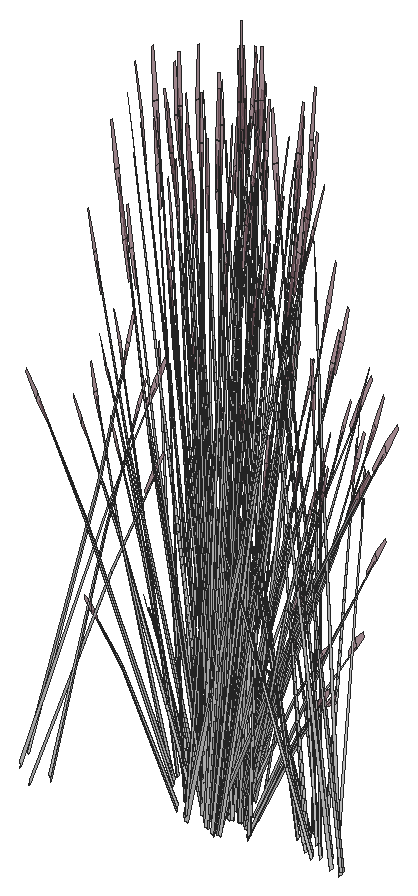
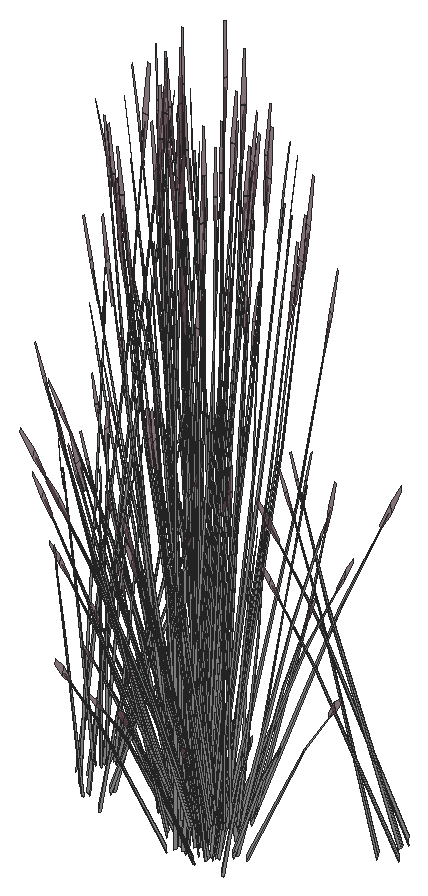
# SketchUp Ruby script. Lengths in inches.
U = 1.inch
M = Sketchup.active_model
def pt(a) = Geom::Point3d.new(a.map { |v| v * U })
def face(e, loops, mat)
  f = e.add_face(loops[0].map { |a| pt(a) })
  loops[1..].each { |l| e.add_face(l.map { |a| pt(a) }).erase! }
  f.material = f.back_material = mat if mat
  f
end
# faces: each face lists its corners as indices into pts; further lists are holes
def faces(e, pts, list, mat = nil) = list.each { |f| face(e, (f[0].is_a?(Array) ? f : [f]).map { |l| l.map { |i| pts[i] } }, mat) }
# xy, xz, yz: faces in a plane at the given z, y or x. An outline is a flat list of corners, or four numbers for a rectangle; further outlines are holes
def ring(l) = l.size == 4 ? [[l[0], l[1]], [l[2], l[1]], [l[2], l[3]], [l[0], l[3]]] : l.each_slice(2).to_a
def flat(e, list, mat, &to3) = list.each { |f| face(e, (f[0].is_a?(Array) ? f : [f]).map { |l| ring(l).map { |u, v| to3.(u, v) } }, mat) }
def xy(e, z, list, mat = nil) = flat(e, list, mat) { |x, y| [x, y, z] }
def xz(e, y, list, mat = nil) = flat(e, list, mat) { |x, z| [x, y, z] }
def yz(e, x, list, mat = nil) = flat(e, list, mat) { |y, z| [x, y, z] }
def lines(e, pts, list) = list.each { |a, b| e.add_line(pt(pts[a]), pt(pts[b])) }
# prism: a flat outline (further loops are holes) pulled along v
def prism(e, loops, v, mat = nil)
  f = face(e, loops, mat); d = Geom::Vector3d.new(v.map { |x| x * U })
  f.pushpull(f.normal.samedirection?(d) ? d.length : -d.length)
end
def box(e, o, s, mat = nil) = prism(e, [[o, [o[0] + s[0], o[1], o[2]], [o[0] + s[0], o[1] + s[1], o[2]], [o[0], o[1] + s[1], o[2]]]], [0, 0, s[2]], mat)
def at(x, y, z, deg = 0) = Geom::Transformation.translation(pt([x, y, z])) * Geom::Transformation.rotation(ORIGIN, Z_AXIS, deg.degrees)
def axes(o, x, y, z) = Geom::Transformation.new([*x, 0, *y, 0, *z, 0, *pt(o).to_a, 1])
def part(name) = M.definitions.add(name)
# library, detail: a bought-in or finely detailed component or shape, given as its bounding box
def library(name, o, s) = part(name).tap { |d| box(d.entities, o, s) }
def detail(e, o, s) = box(e.add_group.entities, o, s)
def put(e, d, t, mat = nil) = e.add_instance(d, t).tap { |i| i.material = mat if mat }
def group(e, t, mat = nil) = e.add_group.tap { |g| g.transformation = t; g.material = mat if mat }.entities
root = M.entities
M.materials.add("LightPink_Translucent").color = [144, 107, 117]
M.materials["LightPink_Translucent"].alpha = 0.75
M.materials.add("[_0053_Ivory_]").color = [200, 200, 200]
c1 = part("blade")
p = [[2.15,0.21,22],[0,0.17,0],[0.09,0.45,0],[2.18,0.31,22],[2.29,0.31,22],[0.38,0.45,0],
  [2.48,0.24,33],[2.49,0.24,33],[2.48,0.22,33]]
faces(c1.entities,p,[[0,1,2,3],[4,5,2,3],[6,3,4,7],[8,0,3,6]])
c2 = part("seeds")
p = [[0.3,-0.1,1.38],[-0.01,-0.03,1.59],[-0.01,-0.03,0.03],[0.14,-0.07,-0.07],[0.29,-0.03,3],[0.15,0.01,3.11]]
faces(c2.entities,p,[[0,1,2,3],[1,0,4,5]],"LightPink_Translucent")
c3 = part("blade with seeds")
put(c3.entities,c1,at(0,0,0))
put(c3.entities,c2,axes([2.4,0.25,30.99],[1.5799,-0.05474,1.17369],[-0.12525,1.92788,0.29478],[-0.07173,-0.02425,1.56792]))
put(root,c3,axes([443.95,105.24,129.13],[0,0.62885,0.49651],[-0.67951,0,0],[0,-0.14322,1.57504]),"[_0053_Ivory_]")
put(root,c3,axes([458.43,104.23,129.32],[-0.61322,0.4175,-0.29095],[-0.40778,-0.58992,-0.50002],[-0.1513,-0.05991,1.59708]),"[_0053_Ivory_]")
put(root,c3,axes([448.72,105.38,131.33],[0.16454,-0.57202,-0.51099],[0.56413,0.19607,-0.3958],[0.22713,-0.05245,0.97773]),"[_0053_Ivory_]")
put(root,c3,axes([447.83,103.05,129.03],[0.37973,-0.63014,0],[0.6353,0.35142,-0.51607],[0.14469,0.08004,1.63711]),"[_0053_Ivory_]")
put(root,c3,axes([443.36,104.3,130.53],[0.25192,-0.01424,1.71376],[-0.16712,0.61729,0.13857],[-0.35901,-0.03818,0.73262]),"[_0053_Ivory_]")
put(root,c3,axes([445.56,105.75,128.86],[-0.36485,-0.52782,-0.44739],[0.55265,-0.37168,0.21531],[-0.11807,-0.06531,1.43643]),"[_0053_Ivory_]")
put(root,c3,axes([445.63,105,129.01],[0.26406,0.70318,0.45755],[-0.7545,0.24452,0.17955],[0.00922,-0.12921,1.58856]),"[_0053_Ivory_]")
put(root,c3,axes([434.7,101.25,129.32],[-0.38947,-0.01972,1.0506],[0.25721,-0.41888,0.58006],[0.15386,0.14882,0.8241]),"[_0053_Ivory_]")
put(root,c3,axes([449.33,105.54,128.64],[-0.39118,0.07547,1.41583],[-0.06226,-0.6007,0.08104],[0.27398,-0.09092,0.80566]),"[_0053_Ivory_]")
put(root,c3,axes([450.04,105.01,128.91],[-0.37654,-0.40212,-0.06488],[0.4124,-0.36845,-0.29416],[0.11685,-0.02594,0.97024]),"[_0053_Ivory_]")
put(root,c3,axes([445.5,105.56,129.37],[-0.29468,0.56664,0.44739],[-0.61229,-0.27271,-0.21531],[0,-0.13062,1.43643]),"[_0053_Ivory_]")
put(root,c3,axes([446.58,105.0625,128.86],[0,-0.72763,0],[0.75945,0,0],[0,0,1.79456]),"[_0053_Ivory_]")
put(root,c3,axes([447.5,103.38,129.13],[-0.56842,-0.31443,0.49651],[0.33976,-0.56381,0],[0.12946,0.07161,1.57504]),"[_0053_Ivory_]")
put(root,c3,axes([448.62,105.59,131.63],[0.53369,-0.27773,-0.71045],[0.29743,0.5717,0.08574],[0.25786,-0.06494,1.00501]),"[_0053_Ivory_]")
put(root,c3,axes([445.23,105.95,128.71],[-0.63179,-0.1031,-0.62353],[0.13332,-0.63596,-0.16365],[-0.18854,-0.07706,1.37633]),"[_0053_Ivory_]")
put(root,c3,axes([446.22,104.6,129.01],[-0.50358,0.57069,0.45755],[-0.59827,-0.50377,0.17955],[0.1214,-0.05695,1.58856]),"[_0053_Ivory_]")
put(root,c3,axes([446.77,105.625,128.95],[-0.56493,-0.54126,-0.06131],[0.56528,-0.54159,0],[-0.01973,-0.0189,1.75571]),"[_0053_Ivory_]")
put(root,c3,axes([433.43,100.23,129.24],[0.01072,-0.20846,1.43002],[0.51218,-0.23285,-0.30754],[0.15811,0.2495,0.61141]),"[_0053_Ivory_]")
put(root,c3,axes([457.16,102.92,130],[0.17264,-0.09097,1.77064],[0.05953,0.63516,0.13857],[-0.37394,0.08428,0.63284]),"[_0053_Ivory_]")
put(root,c3,axes([445.35,103.66,129.13],[-0.17545,0.62497,0.17642],[-0.64204,-0.17686,0.35086],[0.11091,-0.00304,1.60407]),"[_0053_Ivory_]")
put(root,c3,axes([445.08,104.17,128.25],[-0.59782,0.25177,1.28929],[-0.19028,-0.72239,0.50096],[0.36709,0.01202,1.46642]),"[_0053_Ivory_]")
put(root,c3,axes([446.6875,104.36,129.27],[0.11717,-0.56122,0.1448],[0.57245,0.09742,-0.41347],[0.10418,0.05763,1.26744]),"[_0053_Ivory_]")
put(root,c3,axes([459.12,104.42,129.12],[-0.59306,-0.50614,-0.25192],[0.49904,-0.56836,0.5513],[-0.1597,0.05921,1.68216]),"[_0053_Ivory_]")
put(root,c3,axes([445.7,105.69,129.01],[0.76764,0.13249,0.45755],[-0.15622,0.74829,0.17955],[-0.11218,-0.07226,1.58856]),"[_0053_Ivory_]")
put(root,c3,axes([449.75,105.15,128.15],[-0.03174,-0.09547,1.76342],[0.22015,-0.55846,-0.26939],[0.22208,-0.00803,0.30037]),"[_0053_Ivory_]")
put(root,c3,axes([443.2,105.05,128.15],[0.0154,0.09911,1.76342],[-0.31051,0.51756,-0.26939],[-0.22056,-0.02609,0.30037]),"[_0053_Ivory_]")
put(root,c3,axes([446.44,104.51,129.37],[-0.36485,-0.52782,0.44739],[0.55265,-0.37168,-0.21531],[0.11807,0.06531,1.43643]),"[_0053_Ivory_]")
put(root,c3,axes([444.56,106.92,128.68],[-0.14267,-0.54795,-0.30978],[0.56663,-0.1556,0.30978],[-0.11423,-0.06319,1.38974]),"[_0053_Ivory_]")
put(root,c3,axes([455.96,103.27,131.33],[-0.16454,0.57202,-0.51099],[-0.56413,-0.19607,-0.3958],[-0.22713,0.05245,0.97773]),"[_0053_Ivory_]")
put(root,c3,axes([457.23,105.72,129.03],[-0.37973,0.63014,0],[-0.6353,-0.35142,-0.51607],[-0.14469,-0.08004,1.63711]),"[_0053_Ivory_]")
put(root,c3,axes([445.29,106.89,129.13],[0.65264,-0.16691,0.17642],[0.16115,0.62115,0.35086],[-0.05821,-0.0905,1.60407]),"[_0053_Ivory_]")
put(root,c3,axes([446.63,104.54,129.32],[0.61322,-0.4175,-0.29095],[0.40778,0.58992,-0.50002],[0.1513,0.05991,1.59708]),"[_0053_Ivory_]")
put(root,c3,axes([449.07,105.64,131.18],[0.50475,0.17543,-0.35414],[-0.14722,0.5118,0.4572],[0.20322,-0.04693,0.87481]),"[_0053_Ivory_]")
put(root,c3,axes([432.55,100.94,131.33],[0.59704,0.15764,-0.51099],[-0.20464,0.54049,-0.3958],[0.05475,0.21761,0.97773]),"[_0053_Ivory_]")
put(root,c3,axes([432.88,99.82,130.53],[-0.13883,-0.2019,1.71376],[0.64153,-0.16998,0.13857],[0.14499,0.31697,0.73262]),"[_0053_Ivory_]")
put(root,c3,axes([444.4,107.15,128.67],[-0.56842,-0.31443,-0.49651],[0.33976,-0.56381,0],[-0.12946,-0.07161,1.57504]),"[_0053_Ivory_]")
put(root,c3,axes([448.18,103.43,128.67],[0.56842,0.31443,-0.49651],[-0.33976,0.56381,0],[0.12946,0.07161,1.57504]),"[_0053_Ivory_]")
put(root,c3,axes([443.14,104.83,131.18],[-0.50475,-0.17543,-0.35414],[0.14722,-0.5118,0.4572],[-0.20322,0.04693,0.87481]),"[_0053_Ivory_]")
put(root,c3,axes([447.1,105.23,128.86],[0.67951,0,0],[0,0.65103,0],[0,0,1.78407]),"[_0053_Ivory_]")
put(root,c3,axes([445.95,106.04,129.32],[-0.61322,0.4175,-0.29095],[-0.40778,-0.58992,-0.50002],[-0.1513,-0.05991,1.59708]),"[_0053_Ivory_]")
put(root,c3,axes([447.29,103.7,129.13],[-0.65264,0.16691,0.17642],[-0.16115,-0.62115,0.35086],[0.05821,0.0905,1.60407]),"[_0053_Ivory_]")
put(root,c3,axes([447.69,105.01,130.53],[-0.25192,0.01424,1.71376],[0.16712,-0.61729,0.13857],[0.35901,0.03818,0.73262]),"[_0053_Ivory_]")
put(root,c3,axes([448.02,103.67,128.68],[0.14267,0.54795,-0.30978],[-0.56663,0.1556,0.30978],[0.11423,0.06319,1.38974]),"[_0053_Ivory_]")
put(root,c3,axes([446.88,104.89,129.03],[-0.76764,-0.13249,0.49198],[0.15622,-0.74829,0.19306],[0.11218,0.07226,1.70813]),"[_0053_Ivory_]")
put(root,c3,axes([446.27,106.74,128.86],[-0.19817,-0.54216,0],[0.56587,-0.18986,0],[0,0,1.54371]),"[_0053_Ivory_]")
put(root,c3,axes([445.89,106.23,129.27],[-0.11717,0.56122,0.1448],[-0.57245,-0.09742,-0.41347],[-0.10418,-0.05763,1.26744]),"[_0053_Ivory_]")
put(root,c3,axes([455.94,103.5625,130.53],[0.21074,-0.13302,1.71376],[0.17741,0.61464,0.13857],[-0.33083,0.13891,0.73262]),"[_0053_Ivory_]")
put(root,c3,axes([447.01,106.66,128.84],[0.63764,-0.21337,-0.19198],[0.22406,0.61462,0.00008],[0.07038,-0.02358,1.73897]),"[_0053_Ivory_]")
put(root,c3,axes([447.23,106.92,129.13],[0.17545,-0.62497,0.17642],[0.64204,0.17686,0.35086],[-0.11091,0.00304,1.60407]),"[_0053_Ivory_]")
put(root,c3,axes([447.08,105.5,128.87],[0.42396,0.40619,0],[-0.42396,0.40619,0],[0,0,1.69266]),"[_0053_Ivory_]")
put(root,c3,axes([444.67,104.74,130],[0.17264,-0.09097,1.77064],[0.05953,0.63516,0.13857],[-0.37394,0.08428,0.63284]),"[_0053_Ivory_]")
put(root,c3,axes([448.23,105.33,129.13],[-0.47719,-0.45806,0.17642],[0.48088,-0.44429,0.35086],[-0.0527,0.09355,1.60407]),"[_0053_Ivory_]")
put(root,c3,axes([447.35,104.64,128.71],[0.63179,0.1031,-0.62353],[-0.13332,0.63596,-0.16365],[0.18854,0.07706,1.37633]),"[_0053_Ivory_]")
put(root,c3,axes([450.14,105.75,129.42],[-0.37526,0.10382,1.1486],[0.17664,-0.42906,0.84392],[0.19907,0.02936,0.25299]),"[_0053_Ivory_]")
put(root,c3,axes([446.125,106.99,128.85],[-0.61229,-0.28233,0],[0.29468,-0.58663,0],[0,0,1.62707]),"[_0053_Ivory_]")
put(root,c3,axes([446.64,106.23,129.12],[-0.59306,-0.50614,-0.25192],[0.49904,-0.56836,0.5513],[-0.1597,0.05921,1.68216]),"[_0053_Ivory_]")
put(root,c3,axes([445.07,107.2,129.13],[0.56842,0.31443,0.49651],[-0.33976,0.56381,0],[-0.12946,-0.07161,1.57504]),"[_0053_Ivory_]")
put(root,c3,axes([455.29,104.61,129.24],[0.21107,0.05162,1.43002],[0.13604,0.52729,-0.30754],[-0.28671,0.0987,0.61141]),"[_0053_Ivory_]")
put(root,c3,axes([447.08,105.03,129.37],[0.29468,-0.56664,0.44739],[0.61229,0.27271,-0.21531],[0,0.13062,1.43643]),"[_0053_Ivory_]")
put(root,c3,axes([446.96,105.35,128.95],[0,0.72727,-0.05637],[-0.75945,0,0],[0,0.02286,1.79368]),"[_0053_Ivory_]")
put(root,c3,axes([443.48,105.09,131.33],[-0.16454,0.57202,-0.51099],[-0.56413,-0.19607,-0.3958],[-0.22713,0.05245,0.97773]),"[_0053_Ivory_]")
put(root,c3,axes([447.02,104.84,128.86],[0.36485,0.52782,-0.44739],[-0.55265,0.37168,0.21531],[0.11807,0.06531,1.43643]),"[_0053_Ivory_]")
put(root,c3,axes([454.85,105.72,129.42],[0.25312,-0.28501,1.1486],[0.09988,0.45119,0.84392],[-0.18292,0.08079,0.25299]),"[_0053_Ivory_]")
put(root,c3,axes([449.49,107.07,130.58],[-0.11624,-0.52862,-0.03492],[0.54943,-0.12153,-0.15832],[0.11473,0.03351,0.52218]),"[_0053_Ivory_]")
put(root,c3,axes([444.75,107.53,129.03],[-0.37973,0.63014,0],[-0.6353,-0.35142,-0.51607],[-0.14469,-0.08004,1.63711]),"[_0053_Ivory_]")
put(root,c3,axes([455.8,104.48,131.18],[-0.52868,0.08987,-0.35414],[-0.1396,-0.51376,0.4572],[-0.1515,0.13799,0.87481]),"[_0053_Ivory_]")
put(root,c3,axes([448.625,105.34,129.13],[0,-0.62885,0.49651],[0.67951,0,0],[0,0.14322,1.57504]),"[_0053_Ivory_]")
put(root,c3,axes([446.92,105.82,129.37],[0.65953,-0.03882,0.44739],[0.05964,0.64439,-0.21531],[-0.11807,0.06531,1.43643]),"[_0053_Ivory_]")
put(root,c3,axes([447.33,105.16,129.27],[0.56587,-0.18339,0.1448],[0.19817,0.52368,-0.41347],[0,0.11525,1.26744]),"[_0053_Ivory_]")
put(root,c3,axes([446.33,106.13,128.86],[-0.65953,0.03882,-0.44739],[-0.05964,-0.64439,0.21531],[-0.11807,0.06531,1.43643]),"[_0053_Ivory_]")
put(root,c3,axes([449.4375,106.43,129.24],[-0.14627,-0.15466,1.43002],[0.19032,-0.51164,-0.30754],[0.29594,0.06931,0.61141]),"[_0053_Ivory_]")
put(root,c3,axes([458.84,104.68,128.71],[-0.40909,0.47266,-0.62353],[-0.50819,-0.4286,-0.16365],[-0.16393,0.11791,1.37633]),"[_0053_Ivory_]")
put(root,c3,axes([446.82,107,128.86],[0.61229,0.28233,0],[-0.29468,0.58663,0],[0,0,1.74954]),"[_0053_Ivory_]")
put(root,c3,axes([447.07,107.62,128.85],[-0.37499,-0.63235,-0.05142],[0.6353,-0.35142,0.51607],[-0.15655,0.0602,1.6363]),"[_0053_Ivory_]")
put(root,c3,axes([446.93,106.09,129.27],[0.44871,0.37783,0.1448],[-0.37428,0.42627,-0.41347],[-0.10418,0.05763,1.26744]),"[_0053_Ivory_]")
put(root,c3,axes([443.46,105.38,130.53],[0.21074,-0.13302,1.71376],[0.17741,0.61464,0.13857],[-0.33083,0.13891,0.73262]),"[_0053_Ivory_]")
put(root,c3,axes([456.72,103.98,130.53],[0.1517,-0.19322,1.71376],[0.38303,0.52154,0.13857],[-0.26271,0.23751,0.73262]),"[_0053_Ivory_]")
put(root,c3,axes([448.09,106.75,131.63],[0.60713,0.01514,-0.71045],[-0.04078,0.63759,0.08574],[0.25721,0.06729,1.00501]),"[_0053_Ivory_]")
put(root,c3,axes([456.24,104.54,131.33],[0.15602,0.5742,-0.51099],[-0.59087,0.10045,-0.3958],[-0.16933,0.15423,0.97773]),"[_0053_Ivory_]")
put(root,c3,axes([447.41,107.26,129.13],[0.56842,-0.31443,0.49651],[0.33976,0.56381,0],[-0.12946,0.07161,1.57504]),"[_0053_Ivory_]")
put(root,c3,axes([446.6,106.76,128.94],[0.26406,0.72244,-0.06012],[-0.7545,0.25315,0],[0.00922,0.02523,1.72173]),"[_0053_Ivory_]")
put(root,c3,axes([446.89,107.54,128.68],[-0.56663,-0.1556,-0.30978],[0.14267,-0.54795,0.30978],[-0.11423,0.06319,1.38974]),"[_0053_Ivory_]")
put(root,c3,axes([442.81,106.43,129.24],[0.21107,0.05162,1.43002],[0.13604,0.52729,-0.30754],[-0.28671,0.0987,0.61141]),"[_0053_Ivory_]")
put(root,c3,axes([455.51,106.01,128.15],[0.08147,0.06283,1.76342],[0.13814,0.58211,-0.26939],[-0.18056,0.12413,0.30037]),"[_0053_Ivory_]")
put(root,c3,axes([449.09,105.45,129.03],[0.75945,0,0],[0,0.70283,-0.51607],[0,0.16007,1.63711]),"[_0053_Ivory_]")
put(root,c3,axes([448.78,105.8125,128.85],[-0.75908,-0.00503,-0.04976],[0,-0.70283,0.49943],[-0.02386,0.16,1.58352]),"[_0053_Ivory_]")
put(root,c3,axes([447.14,105.2,129.32],[0.68399,0.30005,-0.29095],[-0.32934,0.63331,-0.50002],[0.0215,0.15549,1.59708]),"[_0053_Ivory_]")
put(root,c3,axes([442.37,107.53,129.42],[0.25312,-0.28501,1.1486],[0.09988,0.45119,0.84392],[-0.18292,0.08079,0.25299]),"[_0053_Ivory_]")
put(root,c3,axes([448.46,107.01,131.18],[0.34557,0.39372,-0.35414],[-0.39459,0.37271,0.4572],[0.20048,0.05671,0.87481]),"[_0053_Ivory_]")
put(root,c3,axes([448.625,105.91,128.68],[-0.42396,0.39235,-0.30978],[-0.42396,-0.39235,0.30978],[0,0.12637,1.38974]),"[_0053_Ivory_]")
put(root,c3,axes([446.8,105.95,129.32],[0.07077,0.71755,-0.29095],[-0.73712,0.04339,-0.50002],[-0.1298,0.09558,1.59708]),"[_0053_Ivory_]")
put(root,c3,axes([447.07,105.67,128.86],[-0.29468,0.56664,-0.44739],[-0.61229,-0.27271,0.21531],[0,0.13062,1.43643]),"[_0053_Ivory_]")
put(root,c3,axes([443.32,106.3,131.18],[-0.52868,0.08987,-0.35414],[-0.1396,-0.51376,0.4572],[-0.1515,0.13799,0.87481]),"[_0053_Ivory_]")
put(root,c3,axes([446.35,106.5,128.71],[-0.40909,0.47266,-0.62353],[-0.50819,-0.4286,-0.16365],[-0.16393,0.11791,1.37633]),"[_0053_Ivory_]")
put(root,c3,axes([456.6,104.45,130.53],[0.11309,-0.21615,1.71376],[0.47441,0.44731,0.13857],[-0.21402,0.27879,0.73262]),"[_0053_Ivory_]")
put(root,c3,axes([447.08,107.3,128.98],[0.76036,0.2044,0.30756],[-0.19023,0.7306,-0.36492],[-0.12585,0.09144,1.64885]),"[_0053_Ivory_]")
put(root,c3,axes([447.03,107.79,128.67],[-0.56842,0.31443,-0.49651],[-0.33976,-0.56381,0],[-0.12946,0.07161,1.57504]),"[_0053_Ivory_]")
put(root,c3,axes([448.92,105.93,128.67],[0,0.62885,-0.49651],[-0.67951,0,0],[0,0.14322,1.57504]),"[_0053_Ivory_]")
put(root,c3,axes([447.22,106,130.53],[-0.2256,-0.10835,1.71376],[0.46687,-0.45453,0.13857],[0.29098,0.20505,0.73262]),"[_0053_Ivory_]")
put(root,c3,axes([456.73,105.67,131.18],[-0.41095,0.33109,-0.35414],[-0.38901,-0.37805,0.4572],[-0.05919,0.19208,0.87481]),"[_0053_Ivory_]")
put(root,c3,axes([448.05,107.23,129.42],[-0.34197,-0.18082,1.1486],[0.44156,-0.18372,0.84392],[0.1191,0.15563,0.25299]),"[_0053_Ivory_]")
put(root,c3,axes([444.23,105.8,130.53],[0.1517,-0.19322,1.71376],[0.38303,0.52154,0.13857],[-0.26271,0.23751,0.73262]),"[_0053_Ivory_]")
put(root,c3,axes([443.76,106.36,131.33],[0.15602,0.5742,-0.51099],[-0.59087,0.10045,-0.3958],[-0.16933,0.15423,0.97773]),"[_0053_Ivory_]")
put(root,c3,axes([447.54,107.69,129.03],[0.37973,0.63014,0],[-0.6353,0.35142,-0.51607],[-0.14469,0.08004,1.63711]),"[_0053_Ivory_]")
put(root,c3,axes([448.15,107.9,128.15],[0.04425,-0.09079,1.76342],[0.55709,-0.26738,-0.26939],[0.16889,0.13839,0.30037]),"[_0053_Ivory_]")
put(root,c3,axes([447.22,105.2,129.5],[-0.01659,-0.59209,1.41272],[0.75089,0.15348,0.59816],[-0.1776,0.32398,1.3335]),"[_0053_Ivory_]")
put(root,c3,axes([447.41,105.84,128.75],[0.2227,0.57576,-0.69212],[-0.64151,0.20736,-0.18165],[0.02462,0.19497,1.52773]),"[_0053_Ivory_]")
put(root,c3,axes([443.03,107.83,128.15],[0.08147,0.06283,1.76342],[0.13814,0.58211,-0.26939],[-0.18056,0.12413,0.30037]),"[_0053_Ivory_]")
put(root,c3,axes([447.28,107.48,131.33],[0.59932,-0.14948,-0.51099],[0.10484,0.56611,-0.3958],[0.16097,0.16223,0.97773]),"[_0053_Ivory_]")
put(root,c3,axes([448.11,108.06,129.32],[-0.38947,-0.01972,1.0506],[0.25721,-0.41888,0.58006],[0.15386,0.14882,0.8241]),"[_0053_Ivory_]")
put(root,c3,axes([444.12,106.27,130.53],[0.11309,-0.21615,1.71376],[0.47441,0.44731,0.13857],[-0.21402,0.27879,0.73262]),"[_0053_Ivory_]")
put(root,c3,axes([446.84,107.04,129.24],[0.01072,-0.20846,1.43002],[0.51218,-0.23285,-0.30754],[0.15811,0.2495,0.61141]),"[_0053_Ivory_]")
put(root,c3,axes([456.54,106.63,129.24],[0.19166,-0.0992,1.43002],[0.4732,0.29912,-0.30754],[-0.14084,0.25882,0.61141]),"[_0053_Ivory_]")
put(root,c3,axes([444.25,107.49,131.18],[-0.41095,0.33109,-0.35414],[-0.38901,-0.37805,0.4572],[-0.05919,0.19208,0.87481]),"[_0053_Ivory_]")
put(root,c3,axes([444.51,108.78,129.42],[-0.01572,-0.37392,1.1486],[0.39276,0.26669,0.84392],[-0.07724,0.17822,0.25299]),"[_0053_Ivory_]")
put(root,c3,axes([445.55,107.88,128.15],[0.09829,-0.03422,1.76342],[0.59126,0.18834,-0.26939],[0.01729,0.21228,0.30037]),"[_0053_Ivory_]")
put(root,c3,axes([444.66,107.34,131.66],[0.43478,0.42253,-0.5672],[-0.45929,0.37004,-0.43934],[-0.06615,0.21468,1.08528]),"[_0053_Ivory_]")
put(root,c3,axes([444.1875,107.97,129.48],[0.55175,-0.11136,0.06507],[0.12684,0.44864,-0.86304],[-0.03498,0.22711,0.7736]),"[_0053_Ivory_]")
put(root,c3,axes([445.95,107.74,131.33],[0.59704,0.15764,-0.51099],[-0.20464,0.54049,-0.3958],[0.05475,0.21761,0.97773]),"[_0053_Ivory_]")
put(root,c3,axes([446.29,106.63,130.53],[-0.13883,-0.2019,1.71376],[0.64153,-0.16998,0.13857],[0.14499,0.31697,0.73262]),"[_0053_Ivory_]")
put(root,c3,axes([445.68,108.08,131.18],[-0.1831,0.48359,-0.35414],[-0.53419,-0.14105,0.4572],[0.04898,0.1947,0.87481]),"[_0053_Ivory_]")
put(root,c3,axes([444.52,107.14,131.99],[-0.0158,0.58168,-0.7886],[-0.66548,-0.03907,0.09517],[-0.07023,0.24643,1.11556]),"[_0053_Ivory_]")
put(root,c3,axes([445.15,106.73,130.53],[-0.01487,-0.24136,1.71376],[0.64429,0.16012,0.13857],[-0.03985,0.34396,0.73262]),"[_0053_Ivory_]")
put(root,c3,axes([445.73,107.64,131.63],[0.28988,0.51132,-0.71045],[-0.59671,0.28496,0.08574],[0.06778,0.24706,1.00501]),"[_0053_Ivory_]")
put(root,c3,axes([444.05,108.45,129.24],[0.19166,-0.0992,1.43002],[0.4732,0.29912,-0.30754],[-0.14084,0.25882,0.61141]),"[_0053_Ivory_]")
put(root,c3,axes([444.3,107.96,130.02],[0.01334,-0.32463,1.54345],[0.60018,0.17147,0.21329],[-0.052,0.34598,0.72882]),"[_0053_Ivory_]")
